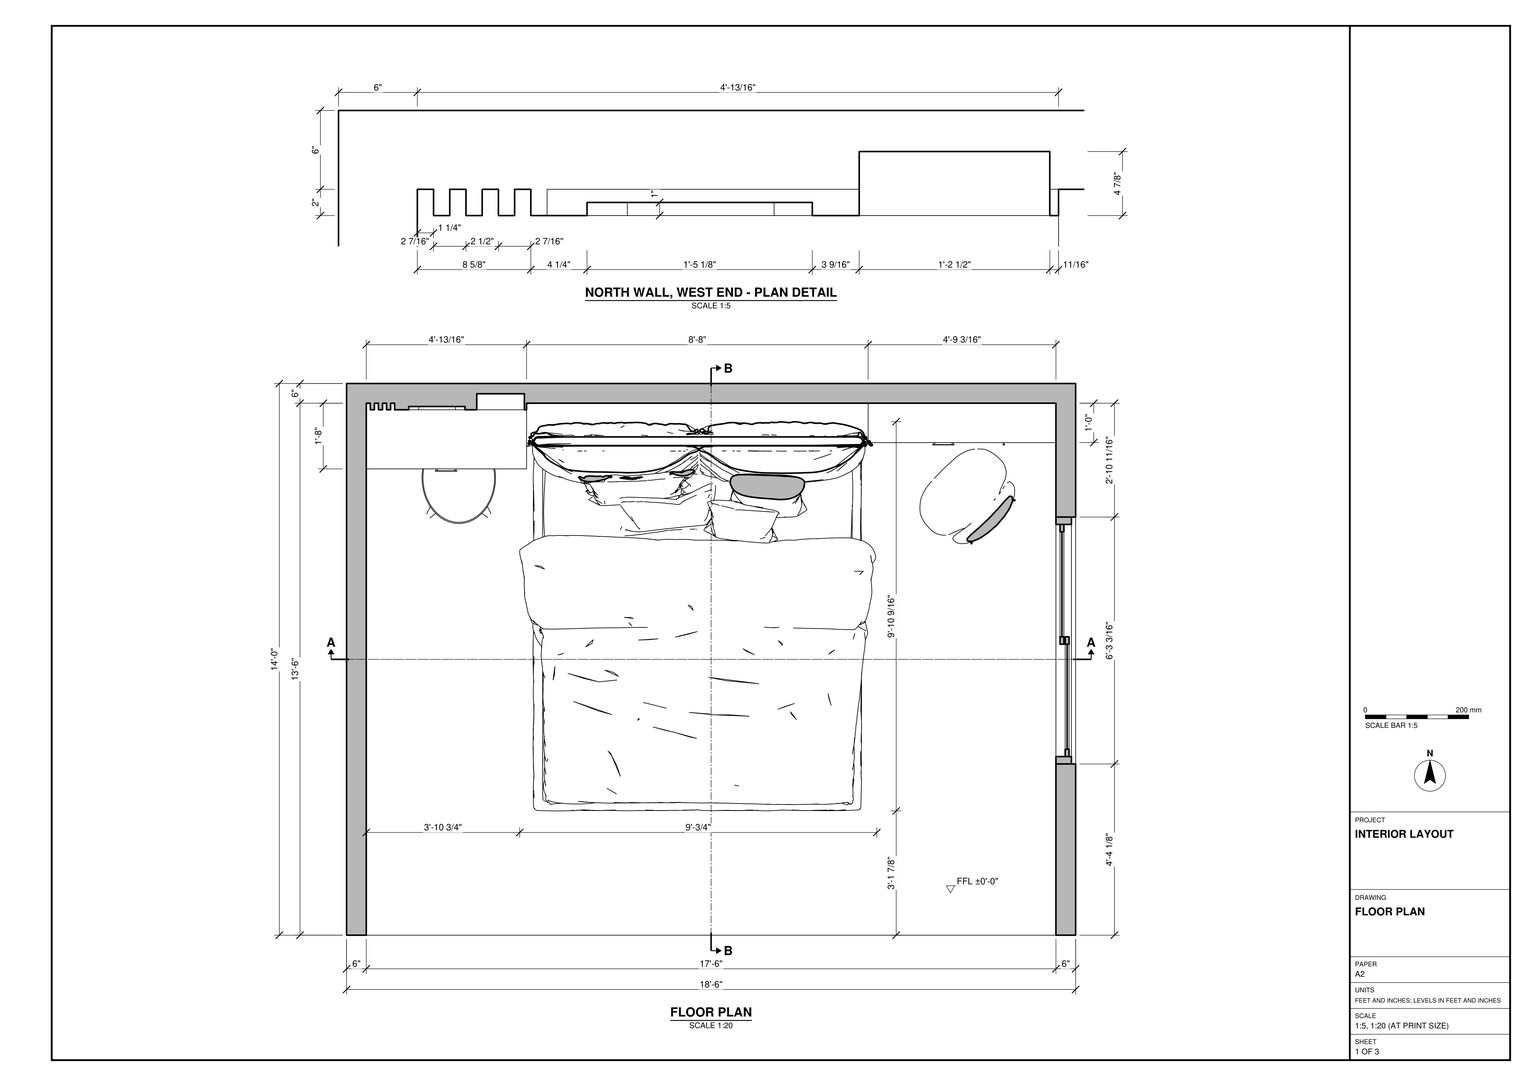
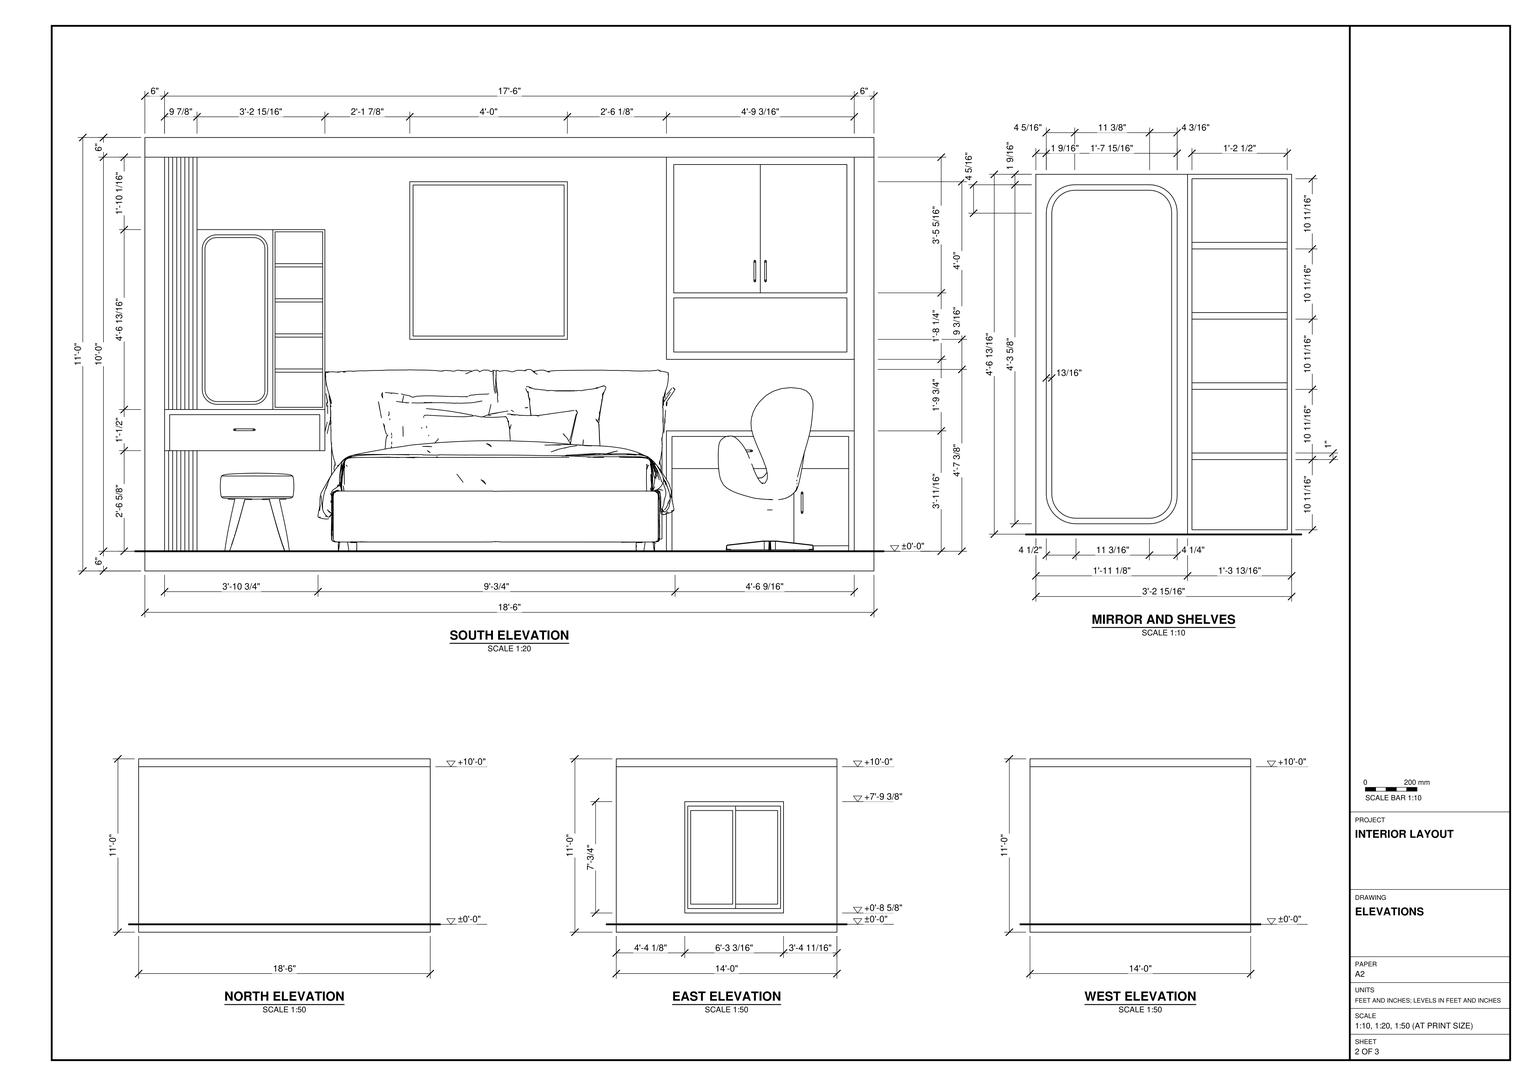
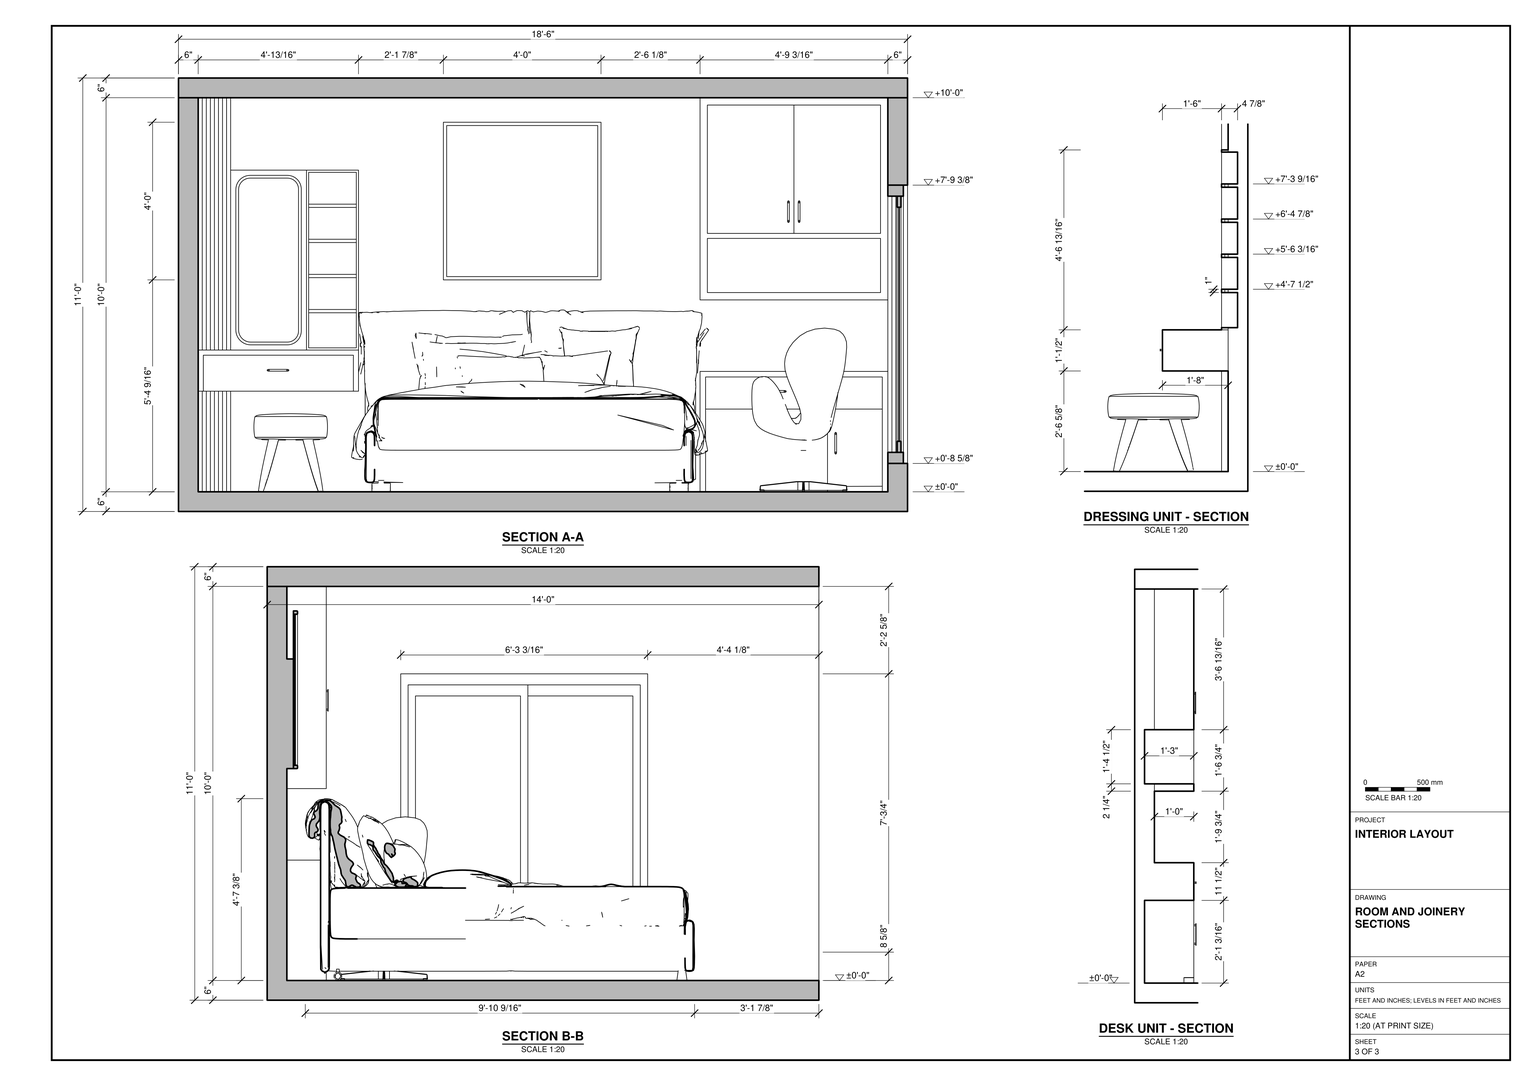
Build the bedroom in SketchUp from task_files/diagram_01.pdf. Work in feet and inches. The room shell measures 18'-6" east to west by 14'-0" north to south and 11'-0" high. Set the finished floor at ±0'-0". Model the 6" north, east and west walls, the 6" floor slab and the 6" ceiling slab, leaving the south side open as shown. Fit the two-panel window into the east wall at the sill height shown in section.

Place the bed with its headboard against the north wall and its foot toward the open side. Use the plan to size the bed and preserve the clear space at its foot. Place the framed artwork above the headboard. At the west end of the north wall, model the vertical slats, floating dressing drawer, rounded-corner mirror and adjacent open shelves. Place the stool in front of the drawer. At the east end, model the desk with knee space, a lower cupboard and wall-mounted storage above. Use the joinery sections to match the depths and vertical spacing, and position the desk chair as shown in plan.

Keep the walls and slabs and each furniture or joinery piece in separate groups or components. Use components for repeated parts. Decor and loose items may be any suitable library components placed as shown. Save one SketchUp model as output_files/bedroom_with_a_dressing_unit_and_built_in_desk.skp.

# SketchUp Ruby script. Lengths in inches.
U = 1.inch
M = Sketchup.active_model
def pt(a) = Geom::Point3d.new(a.map { |v| v * U })
def face(e, loops, mat)
  f = e.add_face(loops[0].map { |a| pt(a) })
  loops[1..].each { |l| e.add_face(l.map { |a| pt(a) }).erase! }
  f.material = f.back_material = mat if mat
  f
end
# faces: each face lists its corners as indices into pts; further lists are holes
def faces(e, pts, list, mat = nil) = list.each { |f| face(e, (f[0].is_a?(Array) ? f : [f]).map { |l| l.map { |i| pts[i] } }, mat) }
# xy, xz, yz: faces in a plane at the given z, y or x. An outline is a flat list of corners, or four numbers for a rectangle; further outlines are holes
def ring(l) = l.size == 4 ? [[l[0], l[1]], [l[2], l[1]], [l[2], l[3]], [l[0], l[3]]] : l.each_slice(2).to_a
def flat(e, list, mat, &to3) = list.each { |f| face(e, (f[0].is_a?(Array) ? f : [f]).map { |l| ring(l).map { |u, v| to3.(u, v) } }, mat) }
def xy(e, z, list, mat = nil) = flat(e, list, mat) { |x, y| [x, y, z] }
def xz(e, y, list, mat = nil) = flat(e, list, mat) { |x, z| [x, y, z] }
def yz(e, x, list, mat = nil) = flat(e, list, mat) { |y, z| [x, y, z] }
def lines(e, pts, list) = list.each { |a, b| e.add_line(pt(pts[a]), pt(pts[b])) }
# prism: a flat outline (further loops are holes) pulled along v
def prism(e, loops, v, mat = nil)
  f = face(e, loops, mat); d = Geom::Vector3d.new(v.map { |x| x * U })
  f.pushpull(f.normal.samedirection?(d) ? d.length : -d.length)
end
def box(e, o, s, mat = nil) = prism(e, [[o, [o[0] + s[0], o[1], o[2]], [o[0] + s[0], o[1] + s[1], o[2]], [o[0], o[1] + s[1], o[2]]]], [0, 0, s[2]], mat)
def at(x, y, z, deg = 0) = Geom::Transformation.translation(pt([x, y, z])) * Geom::Transformation.rotation(ORIGIN, Z_AXIS, deg.degrees)
def axes(o, x, y, z) = Geom::Transformation.new([*x, 0, *y, 0, *z, 0, *pt(o).to_a, 1])
def part(name) = M.definitions.add(name)
# library, detail: a bought-in or finely detailed component or shape, given as its bounding box
def library(name, o, s) = part(name).tap { |d| box(d.entities, o, s) }
def detail(e, o, s) = box(e.add_group.entities, o, s)
def put(e, d, t, mat = nil) = e.add_instance(d, t).tap { |i| i.material = mat if mat }
def group(e, t, mat = nil) = e.add_group.tap { |g| g.transformation = t; g.material = mat if mat }.entities
root = M.entities
M.materials.add("0136_Charcoal metal").color = [35, 35, 35]
M.materials.add("Chrome_Satin1").color = [74, 74, 74]
M.materials.add("Material__1").color = [181, 181, 181]
M.materials.add("Material__2").color = [155, 145, 137]
M.materials.add("Screenshot 2022-04-16 114532").color = [181, 180, 175]
M.materials.add("[0052_FloralWhite]").color = [255, 250, 240]
M.materials.add("[Color M09]").color = [0, 0, 0]
M.materials.add("[CoolGray4]").color = [225, 226, 230]
M.materials["[CoolGray4]"].alpha = 0.26
M.materials.add("[Formica Laminate Light]").color = [230, 154, 75]
M.materials.add("[Quartz Light Grey]").color = [251, 251, 252]
M.materials.add("[Translucent Glass Gray]").color = [188, 188, 188]
M.materials["[Translucent Glass Gray]"].alpha = 0.5
c1 = library("Group\#1",[-1182.41,-748.02,489.16],[424.59,1313.26,379.3])
c2 = library("Group\#2",[-1460.29,-1047.83,411.17],[367.92,2009.52,542.71])
c3 = library("Group\#3",[-1371.82,-1008.11,39.41],[2163.63,1895.35,902.58])
c4 = library("Group\#4",[-1294.08,-968.08,-0.03],[2041.96,1812.57,59.68])
c5 = library("Group\#5",[-802.07,-1084.12,168.98],[1559.29,2039.9,411.2])
c6 = library("Group\#8",[-1317.59,-946.95,218.02],[940.86,1771.32,266.93])
c7 = part("Nathalie+BED")
p = [[0,0,0],[1,0,0],[1,1,0]]
lines(c7.entities,p,[[0,1],[1,2],[2,0]])
put(c7.entities,c1,at(0,0,0))
put(c7.entities,c2,at(0,0,0),"[Quartz Light Grey]")
put(c7.entities,c3,at(0,0,0),"[Formica Laminate Light]")
put(c7.entities,c4,at(0,0,0),"Chrome_Satin1")
put(c7.entities,c5,at(0,0,0),"Material__1")
put(c7.entities,c6,at(0,0,0),"Material__2")
c8 = library("CHAIR",[2.23,-0.9375,0],[23.62,30.08,30.71])
c9 = part("建立群組\#33")
prism(c9.entities,[[[0.39,0,0.2],[0.39,0,0.25],[0.37,0,0.3],[0.34,0,0.34],[0.3,0,0.37],[0.25,0,0.39],[0.2,0,0.39],[0.15,0,0.39],[0.1,0,0.37],[0.06,0,0.34],[0.03,0,0.3],[0.01,0,0.25],[0,0,0.2],[0.01,0,0.15],[0.03,0,0.1],[0.06,0,0.06],[0.1,0,0.03],[0.15,0,0.01],[0.2,0,0],[0.25,0,0.01],[0.3,0,0.03],[0.34,0,0.06],[0.37,0,0.1],[0.39,0,0.15]]],[0,0.59,0])
c10 = part("建立群組\#34")
prism(c10.entities,[[[0.5625,0,-2.8],[0.5625,0,0.32],[0.54,0,0.39],[0.51,0,0.45],[0.45,0,0.51],[0.39,0,0.54],[0.32,0,0.5625],[0.24,0,0.5625],[0.17,0,0.54],[0.11,0,0.51],[0.06,0,0.45],[0.02,0,0.39],[0,0,0.32],[0,0,-2.8],[0.02,0,-2.87],[0.06,0,-2.9375],[0.11,0,-2.99],[0.17,0,-3.03],[0.24,0,-3.05],[0.32,0,-3.05],[0.39,0,-3.03],[0.45,0,-2.99],[0.51,0,-2.9375],[0.54,0,-2.87]]],[0,0.12,0])
c11 = part("建立群組\#32")
prism(c11.entities,[[[0.39,0,0.2],[0.39,0,0.25],[0.37,0,0.3],[0.34,0,0.34],[0.3,0,0.37],[0.25,0,0.39],[0.2,0,0.39],[0.15,0,0.39],[0.1,0,0.37],[0.06,0,0.34],[0.03,0,0.3],[0.01,0,0.25],[0,0,0.2],[0.01,0,0.15],[0.03,0,0.1],[0.06,0,0.06],[0.1,0,0.03],[0.15,0,0.01],[0.2,0,0],[0.25,0,0.01],[0.3,0,0.03],[0.34,0,0.06],[0.37,0,0.1],[0.39,0,0.15]]],[0,0.59,0])
c12 = part("元件\#10")
put(c12.entities,c9,at(0.08,0,0.29),"[Color M09]")
put(c12.entities,c10,axes([0,0.59,5.6],[1,0,0],[0,1,0],[0,0,1.84]),"[Color M09]")
put(c12.entities,c11,at(0.08,0,5.96),"[Color M09]")
c13 = part("把手")
put(c13.entities,c12,at(-0.39,-1.87,0))
c14 = library("stool",[-0.68,-0.68,0],[1.36,1.36,1.75])
c15 = part("Window sash")
g1 = group(c15.entities,at(0.98,0,0))
prism(g1,[[[-0.98,0,0],[30.98,0,0],[30.98,0,45.6],[-0.98,0,45.6]],[[29.01,0,43.625],[29.01,0,1.97],[0.98,0,1.97],[0.98,0,43.625]]],[0,1.18,0])
g2 = group(c15.entities,at(1.97,0.59,1.97))
xz(g2,0,[[0,0,28.03,41.66]],"[CoolGray4]")
c16 = part("Sliding window")
put(c16.entities,c15,at(31.97,2.82,1.97))
put(c16.entities,c15,at(1.97,1.25,1.97))
g3 = group(c16.entities,at(0,0,0))
prism(g3,[[[65.9,4.72,0],[0,4.72,0],[0,4.72,49.53],[65.9,4.72,49.53]],[[1.97,4.72,47.5625],[1.97,4.72,1.97],[63.93,4.72,1.97],[63.93,4.72,47.5625]]],[0,-4.72,0])
c17 = part("Painting 03")
g4 = group(c17.entities,at(0,0,0))
xy(g4,0,[[0,0,1,48]],"0136_Charcoal metal")
xy(g4,1,[[0,1,0.5,47]])
xy(g4,1,[[0.5,1,1,47]],"0136_Charcoal metal")
xy(g4,47,[[0,1,0.5,47]])
xy(g4,47,[[0.5,1,1,47]],"0136_Charcoal metal")
xy(g4,48,[[0,0,1,48]],"0136_Charcoal metal")
xz(g4,0,[[0,0,1,48]],"0136_Charcoal metal")
xz(g4,1,[[0,1,0.5,47]])
xz(g4,1,[[0.5,1,1,47]],"0136_Charcoal metal")
xz(g4,47,[[0,1,0.5,47]])
xz(g4,47,[[0.5,1,1,47]],"0136_Charcoal metal")
xz(g4,48,[[0,0,1,48]],"0136_Charcoal metal")
yz(g4,0,[[1,1,47,47]])
yz(g4,0,[[[0,0,48,48],[1,1,47,47]]],"0136_Charcoal metal")
yz(g4,0.5,[[1,1,47,47]],"Screenshot 2022-04-16 114532")
yz(g4,1.25,[[[0.25,0.25,47.75,47.75],[0.75,0.75,47.25,47.25]]],"0136_Charcoal metal")
p = [[1.06,0.01,0.01],[1.06,0.01,47.99],[1,0,48],[1,0,0],[1.06,47.99,0.01],[1,48,0],
  [1.18,0.07,0.07],[1.18,0.07,47.93],[1.125,0.03,47.97],[1.125,0.03,0.03],[1.18,47.93,0.07],[1.125,47.97,0.03],
  [1.18,47.93,47.93],[1.125,47.97,47.97],[1.06,47.99,47.99],[1,48,48],[1.24,0.19,0.19],[1.24,0.19,47.81],
  [1.22,0.125,47.875],[1.22,0.125,0.125],[1.24,47.81,0.19],[1.22,47.875,0.125],[1.24,47.81,47.81],[1.22,47.875,47.875],
  [1.25,0.25,0.25],[1.25,0.25,47.75],[1.25,47.75,0.25],[1.25,47.75,47.75],[1.24,0.81,0.81],[1.24,47.19,0.81],
  [1.22,47.125,0.875],[1.22,0.875,0.875],[1.25,0.75,0.75],[1.25,47.25,0.75],[1.25,0.75,47.25],[1.24,0.81,47.19],
  [1.22,0.875,47.125],[1.24,47.19,47.19],[1.22,47.125,47.125],[1.25,47.25,47.25],[1.18,0.93,0.93],[1.18,47.07,0.93],
  [1.125,47.03,0.97],[1.125,0.97,0.97],[1.18,0.93,47.07],[1.125,0.97,47.03],[1.18,47.07,47.07],[1.125,47.03,47.03],
  [1.06,0.99,0.99],[1.06,47.01,0.99],[1,47,1],[1,1,1],[1.06,0.99,47.01],[1,1,47],
  [1.06,47.01,47.01],[1,47,47]]
faces(g4,p,[[0,1,2,3],[4,0,3,5],[6,7,8,9],[9,8,1,0],[10,6,9,11],[11,9,0,4],[12,10,11,13],[14,4,5,15],
  [13,11,4,14],[16,17,18,19],[20,16,19,21],[19,18,7,6],[21,19,6,10],[22,20,21,23],[23,21,10,12],[24,25,17,16],
  [26,24,16,20],[27,26,20,22],[28,29,30,31],[32,33,29,28],[34,32,28,35],[35,28,31,36],[29,37,38,30],[33,39,37,29],
  [40,41,42,43],[44,40,43,45],[31,30,41,40],[36,31,40,44],[41,46,47,42],[30,38,46,41],[48,49,50,51],[52,48,51,53],
  [45,43,48,52],[43,42,49,48],[49,54,55,50],[42,47,54,49],[46,44,45,47],[54,52,53,55],[47,45,52,54],[37,35,36,38],
  [38,36,44,46],[39,34,35,37],[17,22,23,18],[25,27,22,17],[7,12,13,8],[18,23,12,7],[1,14,15,2],[8,13,14,1]],"0136_Charcoal metal")
box(root,[0,0,126],[222,168,6])
put(root,c7,axes([110.34,79.52,6],[0,-0.05264,0],[0.05314,0,0],[0,0,0.05805]))
put(root,c8,axes([209.44,133.15,6],[-0.70711,0.70711,0],[-0.70711,-0.70711,0],[0,0,1.62325]))
put(root,c13,axes([33.62,140.13,42.9],[0,0,-1],[0,-1,0],[-1,0,0]))
put(root,c13,axes([185.06,148.13,36.47],[0,0,-1],[0,-1,0],[-1,0,0]))
put(root,c13,axes([200.22,148.13,24.12],[1,0,0],[0,-1,0],[0,0,-1]))
put(root,c13,axes([189.09,148.26,94.63],[1,0,0],[0,-1,0],[0,0,-1]))
put(root,c13,axes([185.84,148.26,94.63],[1,0,0],[0,-1,0],[0,0,-1]))
put(root,c14,axes([34.16,139.27,6],[16.554,0,0],[0,20.565,0],[0,0,13.585]))
put(root,c16,axes([216,127.33,14.64],[0,-1.14092,0],[1,0,0],[0,0,1.711]))
put(root,c17,at(80.66,160,70.53,-90))
g5 = group(root,at(0,0,0))
xy(g5,0,[[0,0,222,168]])
xy(g5,6,[[6,0,216,0,216,150,214.31,150,214.31,153,197.63,153,197.63,165,160.5,165,160.5,150,158.8125,150,158.8125,162,15.875,162,15.875,160,14.64,160,14.64,162,13.41,162,13.41,160,12.17,160,12.17,162,10.9375,162,10.9375,160,9.7,160,9.7,162,8.47,162,8.47,160,7.23,160,7.23,162,6,162]])
xy(g5,14.64,[[216,52.14,222,127.33]])
xy(g5,31.1875,[[160.5,150,197.63,165]],"[Formica Laminate Light]")
xy(g5,36.64,[[6,142,6,162,7.23,162,7.23,160,8.47,160,8.47,162,9.7,162,9.7,160,10.9375,160,10.9375,162,12.17,162,12.17,160,13.41,160,13.41,162,14.64,162,14.64,160,15.875,160,15.875,162,54.8125,162,54.8125,142]],"[Formica Laminate Light]")
xy(g5,42.66,[[158.8125,150,216,162]],"[Formica Laminate Light]")
xy(g5,49.16,[[6,142,54.8125,142,54.8125,160,14.64,160,14.64,162,13.41,162,13.41,160,12.17,160,12.17,162,10.9375,162,10.9375,160,9.7,160,9.7,162,8.47,162,8.47,160,7.23,160,7.23,162,6,162]],"[Formica Laminate Light]")
xy(g5,49.83,[[39.64,160,54.15,164.875]],"[Formica Laminate Light]")
xy(g5,51.59,[[21.99,160,33.16,161]],"[Formica Laminate Light]")
xy(g5,60.52,[[39.64,160,54.15,164.875]],"[Formica Laminate Light]")
xy(g5,61.52,[[39.64,160,54.15,164.875]],"[Formica Laminate Light]")
xy(g5,64.4375,[[158.8125,150,216,162]],"[Formica Laminate Light]")
xy(g5,66.67,[[161.04,150,213.77,165]],"[Formica Laminate Light]")
xy(g5,70.53,[[89.85,160,116.66,162]],"[0052_FloralWhite]")
xy(g5,71.21,[[39.64,160,54.15,164.875]],"[Formica Laminate Light]")
xy(g5,72.21,[[39.64,160,54.15,164.875]],"[Formica Laminate Light]")
xy(g5,81.9,[[39.64,160,54.15,164.875]],"[Formica Laminate Light]")
xy(g5,82.9,[[39.64,160,54.15,164.875]],"[Formica Laminate Light]")
xy(g5,83.16,[[161.04,150,213.77,165]],"[Formica Laminate Light]")
xy(g5,92.59,[[39.64,160,54.15,164.875]],"[Formica Laminate Light]")
xy(g5,93.59,[[39.64,160,54.15,164.875]],"[Formica Laminate Light]")
xy(g5,99.39,[[216,52.14,222,127.33]])
xy(g5,101.52,[[21.79,160,33.1875,161]],"[Formica Laminate Light]")
xy(g5,103.28,[[39.64,160,54.15,164.875]],"[Formica Laminate Light]")
xy(g5,103.91,[[89.85,160,116.66,162]],"[0052_FloralWhite]")
xy(g5,103.95,[[15.875,160,54.8125,162]],"[Formica Laminate Light]")
xy(g5,126,[[0,0,6,162],[216,0,222,162]])
xy(g5,126,[[158.8125,150,216,150,216,162,222,162,222,168,0,168,0,162,7.23,162,7.23,160,8.47,160,8.47,162,9.7,162,9.7,160,10.9375,160,10.9375,162,12.17,162,12.17,160,13.41,160,13.41,162,14.64,162,14.64,160,15.875,160,15.875,162,158.8125,162]],"[Formica Laminate Light]")
xz(g5,0,[[0,0,222,0,222,6,6,6,6,126,0,126],[216,6,222,126]])
xz(g5,52.14,[[216,14.64,222,99.39]])
xz(g5,127.33,[[216,14.64,222,99.39]])
xz(g5,142,[[6,36.64,7.56,36.64,7.56,47.6,53.25,47.6,53.25,36.64,54.8125,36.64,54.8125,49.16,6,49.16],[7.56,36.64,53.25,47.6]],"[Formica Laminate Light]")
xz(g5,150,[[158.8125,6,160.5,6,160.5,40.97,214.31,40.97,214.31,6,216,6,216,42.66,158.8125,42.66],[197.63,7.63,214.31,7.69,214.31,31.1875,197.63,31.1875],[160.5,31.1875,214.31,40.97],[[158.8125,64.4375,216,126],[161.04,84.6875,213.77,123.77],[161.04,66.67,213.77,83.16]],[161.04,84.6875,187.41,123.77],
  [187.41,84.6875,213.77,123.77]],"[Formica Laminate Light]")
xz(g5,153,[[197.63,6,214.31,6,214.31,7.69,197.63,7.63]],"[Formica Laminate Light]")
xz(g5,160,[[89.85,70.53,116.66,103.91]],"[0052_FloralWhite]")
xz(g5,160,[[7.23,6,8.47,36.64],[9.7,6,10.9375,36.64],[12.17,6,13.41,36.64],[14.64,6,15.875,36.64],[7.23,49.16,8.47,126],
  [9.7,49.16,10.9375,126],[12.17,49.16,13.41,126],[14.64,49.16,15.875,126],[[15.875,49.16,38.97,103.95],[21.99,50.75,21.4,50.78,20.82,50.9,20.25,51.09,19.72,51.35,19.23,51.68,18.79,52.07,18.4,52.52,18.07,53.01,17.81,53.54,17.62,54.1,17.5,54.68,17.46,55.27,17.46,98.03,17.5,98.6,17.61,99.15,17.79,99.6875,18.04,100.2,18.36,100.67,18.73,101.09,19.16,101.47,19.625,101.78,20.13,102.03,20.67,102.21,21.23,102.33,21.79,102.36,33.1875,102.36,33.73,102.33,34.27,102.22,34.79,102.04,35.29,101.8,35.74,101.49,36.16,101.13,36.52,100.72,36.82,100.26,37.07,99.77,37.24,99.25,37.35,98.71,37.39,98.16,37.39,54.97,37.35,54.42,37.24,53.88,37.0625,53.35,36.82,52.86,36.51,52.4,36.15,51.98,35.73,51.62,35.27,51.3125,34.78,51.07,34.25,50.89,33.71,50.78,33.16,50.75]],[[38.97,49.16,54.8125,103.95],[39.64,49.83,54.15,103.28]],
  [[21.99,50.75,33.16,50.75,33.71,50.78,34.25,50.89,34.78,51.07,35.27,51.3125,35.73,51.62,36.15,51.98,36.51,52.4,36.82,52.86,37.0625,53.35,37.24,53.88,37.35,54.42,37.39,54.97,37.39,98.16,37.35,98.71,37.24,99.25,37.07,99.77,36.82,100.26,36.52,100.72,36.16,101.13,35.74,101.49,35.29,101.8,34.79,102.04,34.27,102.22,33.73,102.33,33.1875,102.36,21.79,102.36,21.23,102.33,20.67,102.21,20.13,102.03,19.625,101.78,19.16,101.47,18.73,101.09,18.36,100.67,18.04,100.2,17.79,99.6875,17.61,99.15,17.5,98.6,17.46,98.03,17.46,55.27,17.5,54.68,17.62,54.1,17.81,53.54,18.07,53.01,18.4,52.52,18.79,52.07,19.23,51.68,19.72,51.35,20.25,51.09,20.82,50.9,21.4,50.78],[21.99,51.59,21.51,51.62,21.03,51.71,20.58,51.87,20.14,52.08,19.74,52.35,19.38,52.67,19.0625,53.03,18.8,53.43,18.58,53.86,18.43,54.32,18.33,54.79,18.3,55.27,18.3,98.03,18.33,98.49,18.42,98.93,18.57,99.37,18.77,99.78,19.02,100.16,19.32,100.5,19.67,100.8,20.05,101.05,20.46,101.26,20.89,101.4,21.34,101.49,21.79,101.52,33.1875,101.52,33.625,101.49,34.06,101.41,34.47,101.27,34.87,101.07,35.23,100.83,35.5625,100.54,35.85,100.21,36.09,99.84,36.29,99.45,36.43,99.03,36.52,98.6,36.54,98.16,36.54,54.97,36.52,54.53,36.43,54.1,36.29,53.68,36.09,53.28,35.85,52.91,35.55,52.58,35.22,52.29,34.85,52.04,34.45,51.84,34.04,51.7,33.6,51.62,33.16,51.59]],[39.64,60.52,54.15,61.52],[39.64,71.21,54.15,72.21],[39.64,81.9,54.15,82.9],[39.64,92.59,54.15,93.59]],"[Formica Laminate Light]")
xz(g5,161,[[21.99,51.59,33.16,51.59,33.6,51.62,34.04,51.7,34.45,51.84,34.85,52.04,35.22,52.29,35.55,52.58,35.85,52.91,36.09,53.28,36.29,53.68,36.43,54.1,36.52,54.53,36.54,54.97,36.54,98.16,36.52,98.6,36.43,99.03,36.29,99.45,36.09,99.84,35.85,100.21,35.5625,100.54,35.23,100.83,34.87,101.07,34.47,101.27,34.06,101.41,33.625,101.49,33.1875,101.52,21.79,101.52,21.34,101.49,20.89,101.4,20.46,101.26,20.05,101.05,19.67,100.8,19.32,100.5,19.02,100.16,18.77,99.78,18.57,99.37,18.42,98.93,18.33,98.49,18.3,98.03,18.3,55.27,18.33,54.79,18.43,54.32,18.58,53.86,18.8,53.43,19.0625,53.03,19.38,52.67,19.74,52.35,20.14,52.08,20.58,51.87,21.03,51.71,21.51,51.62]],"[Translucent Glass Gray]")
xz(g5,162,[[[15.875,6,158.8125,6,158.8125,42.66,216,42.66,216,64.4375,158.8125,64.4375,158.8125,126,15.875,126,15.875,103.95,54.8125,103.95,54.8125,36.64,15.875,36.64],[89.85,70.53,116.66,103.91]]],"[0052_FloralWhite]")
xz(g5,162,[[6,6,7.23,36.64],[8.47,6,9.7,36.64],[10.9375,6,12.17,36.64],[13.41,6,14.64,36.64],[6,49.16,7.23,126],
  [8.47,49.16,9.7,126],[10.9375,49.16,12.17,126],[13.41,49.16,14.64,126]],"[Formica Laminate Light]")
xz(g5,164.875,[[39.64,49.83,54.15,60.52],[39.64,61.52,54.15,71.21],[39.64,72.21,54.15,81.9],[39.64,82.9,54.15,92.59],[39.64,93.59,54.15,103.28]],"[Formica Laminate Light]")
xz(g5,165,[[160.5,6,197.63,31.1875]],"[0052_FloralWhite]")
xz(g5,165,[[161.04,66.67,213.77,83.16]],"[Formica Laminate Light]")
xz(g5,168,[[0,0,222,126]],"[0052_FloralWhite]")
yz(g5,0,[[0,0,168,126]],"[0052_FloralWhite]")
yz(g5,6,[[0,6,162,6,162,36.64,142,36.64,142,49.16,162,49.16,162,126,0,126],[142,36.64,162,49.16]])
yz(g5,6,[[142,36.64,162,49.16]],"[Formica Laminate Light]")
yz(g5,7.23,[[160,6,162,36.64],[160,49.16,162,126]],"[Formica Laminate Light]")
yz(g5,8.47,[[160,6,162,36.64],[160,49.16,162,126]],"[Formica Laminate Light]")
yz(g5,9.7,[[160,6,162,36.64],[160,49.16,162,126]],"[Formica Laminate Light]")
yz(g5,10.9375,[[160,6,162,36.64],[160,49.16,162,126]],"[Formica Laminate Light]")
yz(g5,12.17,[[160,6,162,36.64],[160,49.16,162,126]],"[Formica Laminate Light]")
yz(g5,13.41,[[160,6,162,36.64],[160,49.16,162,126]],"[Formica Laminate Light]")
yz(g5,14.64,[[160,6,162,36.64],[160,49.16,162,126]],"[Formica Laminate Light]")
yz(g5,15.875,[[160,6,162,36.64],[160,103.95,162,126]],"[Formica Laminate Light]")
yz(g5,18.3,[[160,55.27,161,98.03]],"[Formica Laminate Light]")
yz(g5,36.54,[[160,54.97,161,98.16]],"[Formica Laminate Light]")
yz(g5,39.64,[[160,49.83,164.875,60.52],[160,61.52,164.875,71.21],[160,72.21,164.875,81.9],[160,82.9,164.875,92.59],[160,93.59,164.875,103.28]],"[Formica Laminate Light]")
yz(g5,54.15,[[160,49.83,164.875,60.52],[160,61.52,164.875,71.21],[160,72.21,164.875,81.9],[160,82.9,164.875,92.59],[160,93.59,164.875,103.28]],"[Formica Laminate Light]")
yz(g5,54.8125,[[142,36.64,162,36.64,162,103.95,160,103.95,160,49.16,142,49.16]],"[Formica Laminate Light]")
yz(g5,89.85,[[160,70.53,162,103.91]],"[0052_FloralWhite]")
yz(g5,116.66,[[160,70.53,162,103.91]],"[0052_FloralWhite]")
yz(g5,158.8125,[[150,6,162,42.66],[150,64.4375,162,126]],"[Formica Laminate Light]")
yz(g5,160.5,[[150,6,165,31.1875]],"[Formica Laminate Light]")
yz(g5,161.04,[[150,66.67,165,83.16]],"[Formica Laminate Light]")
yz(g5,197.63,[[153,6,153,7.63,150,7.63,150,31.1875,165,31.1875,165,6]],"[Formica Laminate Light]")
yz(g5,213.77,[[150,66.67,165,83.16]],"[Formica Laminate Light]")
yz(g5,214.31,[[150,6,153,7.69]])
yz(g5,216,[[[0,6,0,126,150,126,150,64.4375,162,64.4375,162,42.66,150,42.66,150,6],[52.14,14.64,127.33,99.39]]])
yz(g5,216,[[150,64.4375,162,126]],"[Formica Laminate Light]")
yz(g5,222,[[[0,0,168,126],[52.14,14.64,127.33,99.39]]])
p = [[214.31,150,7.69],[197.63,150,7.63],[197.63,153,7.63],[214.31,153,7.69],[21.03,160,51.71],[21.51,160,51.62],
  [21.51,161,51.62],[21.03,161,51.71],[21.99,160,51.59],[21.99,161,51.59],[33.16,160,51.59],[33.6,160,51.62],
  [33.6,161,51.62],[33.16,161,51.59],[34.04,160,51.7],[34.04,161,51.7],[20.58,160,51.87],[20.58,161,51.87],
  [34.45,160,51.84],[34.45,161,51.84],[34.85,160,52.04],[34.85,161,52.04],[20.14,160,52.08],[20.14,161,52.08],
  [35.22,160,52.29],[35.22,161,52.29],[19.74,160,52.35],[19.74,161,52.35],[19.38,160,52.67],[19.38,161,52.67],
  [35.55,160,52.58],[35.55,161,52.58],[35.85,160,52.91],[35.85,161,52.91],[19.0625,160,53.03],[19.0625,161,53.03],
  [36.09,160,53.28],[36.09,161,53.28],[18.8,160,53.43],[18.8,161,53.43],[36.29,160,53.68],[36.29,161,53.68],
  [18.58,160,53.86],[18.58,161,53.86],[36.43,160,54.1],[36.43,161,54.1],[18.43,160,54.32],[18.43,161,54.32],
  [36.52,160,54.53],[36.52,161,54.53],[18.33,160,54.79],[18.33,161,54.79],[36.54,160,54.97],[36.54,161,54.97],
  [18.3,160,55.27],[18.3,161,55.27],[18.33,160,98.49],[18.3,160,98.03],[18.3,161,98.03],[18.33,161,98.49],
  [36.54,160,98.16],[36.52,160,98.6],[36.52,161,98.6],[36.54,161,98.16],[18.42,160,98.93],[18.42,161,98.93],
  [36.43,160,99.03],[36.43,161,99.03],[18.57,160,99.37],[18.57,161,99.37],[36.29,160,99.45],[36.29,161,99.45],
  [18.77,160,99.78],[18.77,161,99.78],[36.09,160,99.84],[36.09,161,99.84],[19.02,160,100.16],[19.02,161,100.16],
  [35.85,160,100.21],[35.85,161,100.21],[19.32,160,100.5],[19.32,161,100.5],[35.5625,160,100.54],[35.5625,161,100.54],
  [19.67,160,100.8],[19.67,161,100.8],[35.23,160,100.83],[35.23,161,100.83],[20.05,160,101.05],[20.05,161,101.05],
  [34.87,160,101.07],[34.87,161,101.07],[20.46,160,101.26],[20.46,161,101.26],[34.47,160,101.27],[34.47,161,101.27],
  [20.89,160,101.4],[20.89,161,101.4],[34.06,160,101.41],[34.06,161,101.41],[21.34,160,101.49],[21.34,161,101.49],
  [33.625,160,101.49],[33.625,161,101.49],[21.79,160,101.52],[21.79,161,101.52],[33.1875,160,101.52],[33.1875,161,101.52]]
faces(g5,p,[[0,1,2,3],[4,5,6,7],[5,8,9,6],[10,11,12,13],[11,14,15,12],[16,4,7,17],[14,18,19,15],[18,20,21,19],
  [22,16,17,23],[20,24,25,21],[26,22,23,27],[28,26,27,29],[24,30,31,25],[30,32,33,31],[34,28,29,35],[32,36,37,33],
  [38,34,35,39],[36,40,41,37],[42,38,39,43],[40,44,45,41],[46,42,43,47],[44,48,49,45],[50,46,47,51],[48,52,53,49],
  [54,50,51,55],[56,57,58,59],[60,61,62,63],[64,56,59,65],[61,66,67,62],[68,64,65,69],[66,70,71,67],[72,68,69,73],
  [70,74,75,71],[76,72,73,77],[74,78,79,75],[80,76,77,81],[78,82,83,79],[84,80,81,85],[82,86,87,83],[88,84,85,89],
  [86,90,91,87],[92,88,89,93],[90,94,95,91],[96,92,93,97],[94,98,99,95],[100,96,97,101],[98,102,103,99],[104,100,101,105],
  [102,106,107,103]],"[Formica Laminate Light]")
